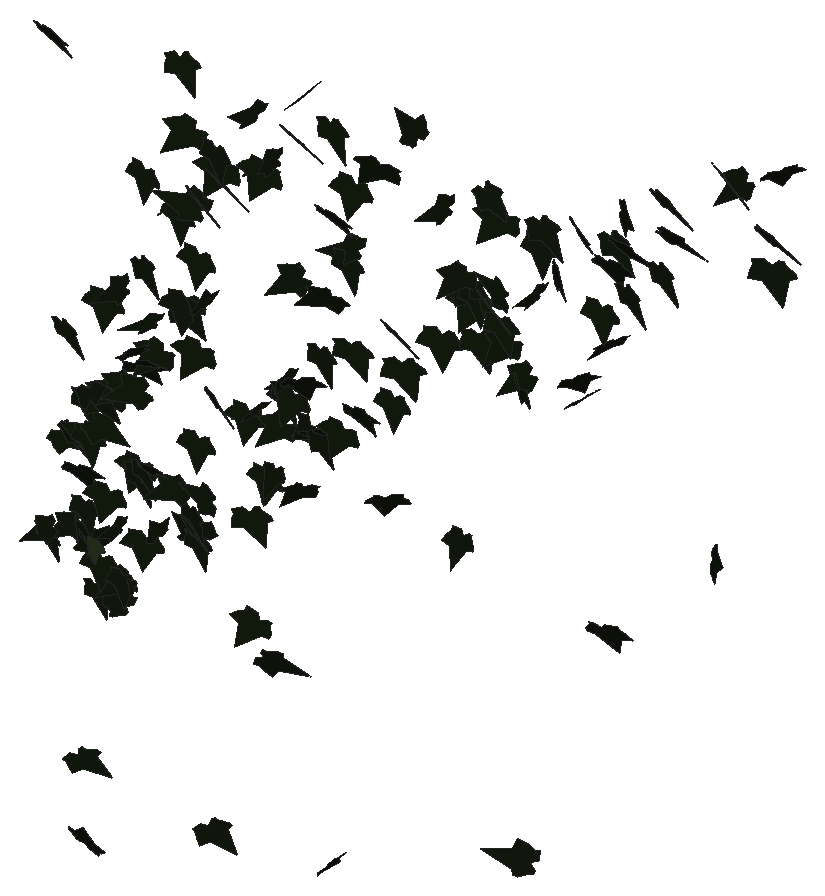
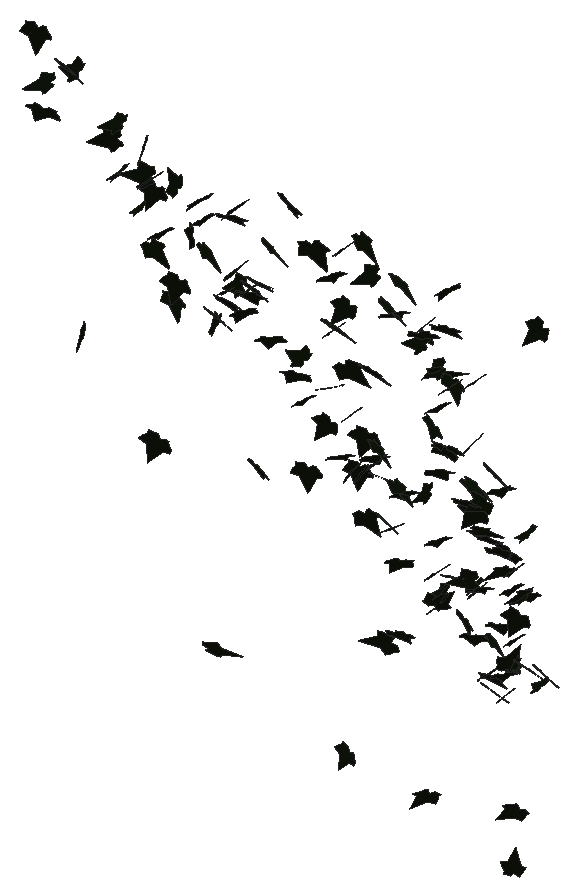
# SketchUp Ruby script. Lengths in inches.
U = 1.inch
M = Sketchup.active_model
def pt(a) = Geom::Point3d.new(a.map { |v| v * U })
def face(e, loops, mat)
  f = e.add_face(loops[0].map { |a| pt(a) })
  loops[1..].each { |l| e.add_face(l.map { |a| pt(a) }).erase! }
  f.material = f.back_material = mat if mat
  f
end
# faces: each face lists its corners as indices into pts; further lists are holes
def faces(e, pts, list, mat = nil) = list.each { |f| face(e, (f[0].is_a?(Array) ? f : [f]).map { |l| l.map { |i| pts[i] } }, mat) }
# xy, xz, yz: faces in a plane at the given z, y or x. An outline is a flat list of corners, or four numbers for a rectangle; further outlines are holes
def ring(l) = l.size == 4 ? [[l[0], l[1]], [l[2], l[1]], [l[2], l[3]], [l[0], l[3]]] : l.each_slice(2).to_a
def flat(e, list, mat, &to3) = list.each { |f| face(e, (f[0].is_a?(Array) ? f : [f]).map { |l| ring(l).map { |u, v| to3.(u, v) } }, mat) }
def xy(e, z, list, mat = nil) = flat(e, list, mat) { |x, y| [x, y, z] }
def xz(e, y, list, mat = nil) = flat(e, list, mat) { |x, z| [x, y, z] }
def yz(e, x, list, mat = nil) = flat(e, list, mat) { |y, z| [x, y, z] }
def lines(e, pts, list) = list.each { |a, b| e.add_line(pt(pts[a]), pt(pts[b])) }
# prism: a flat outline (further loops are holes) pulled along v
def prism(e, loops, v, mat = nil)
  f = face(e, loops, mat); d = Geom::Vector3d.new(v.map { |x| x * U })
  f.pushpull(f.normal.samedirection?(d) ? d.length : -d.length)
end
def box(e, o, s, mat = nil) = prism(e, [[o, [o[0] + s[0], o[1], o[2]], [o[0] + s[0], o[1] + s[1], o[2]], [o[0], o[1] + s[1], o[2]]]], [0, 0, s[2]], mat)
def at(x, y, z, deg = 0) = Geom::Transformation.translation(pt([x, y, z])) * Geom::Transformation.rotation(ORIGIN, Z_AXIS, deg.degrees)
def axes(o, x, y, z) = Geom::Transformation.new([*x, 0, *y, 0, *z, 0, *pt(o).to_a, 1])
def part(name) = M.definitions.add(name)
# library, detail: a bought-in or finely detailed component or shape, given as its bounding box
def library(name, o, s) = part(name).tap { |d| box(d.entities, o, s) }
def detail(e, o, s) = box(e.add_group.entities, o, s)
def put(e, d, t, mat = nil) = e.add_instance(d, t).tap { |i| i.material = mat if mat }
def group(e, t, mat = nil) = e.add_group.tap { |g| g.transformation = t; g.material = mat if mat }.entities
root = M.entities
M.materials.add("1026 AP 7946 SUNNY SIDE UP").color = [254, 231, 186]
M.materials.add("efeu1").color = [18, 25, 13]
M.materials.add("efeu2").color = [43, 57, 29]
c1 = part("ivyleaf_9")
p = [[1.54,2.16,1.25],[1.36,2.04,1.19],[-0.21,0.99,0.68],[-0.71,1.11,0.82],[-0.85,0.86,0.67],[-0.8,0.17,0.21],
  [-0.9,-0.01,0.1],[-0.67,-0.16,-0.02],[-0.08,-0.08,-0.05],[-0.03,-0.6,-0.4],[0.65,-0.88,-0.66],[0.83,-0.6,-0.49],
  [1.29,-0.42,-0.43],[1.8125,-0.07,-0.26],[1.21,0.44,0.15]]
faces(c1.entities,p,[[0,1,2,3,4,5,6,7,8,9,10,11,12,13,14]],"efeu1")
c2 = part("ivyleaf_10")
p = [[0,0.5,-0.03],[-0.0625,2.02,-0.43],[-0.19,2.01,-0.46],[-0.54,1.05,-0.29],[-0.52,0.625,-0.18],[-0.83,0.76,-0.28],
  [-1.16,0.64,-0.33],[-1.15,0.33,-0.24],[-0.77,-0.39,0.02],[-0.3,-0.51,0.16],[0.04,-0.48,0.23],[-0.02,2.01,-0.4375],
  [-0.06,2.01,-0.43],[0.04,-0.49,0.23],[0.67,-0.49,0.14],[1.38,0.36,-0.2],[1.375,0.51,-0.24],[0.81,0.65,-0.19],
  [0.62,0.59,-0.15],[0.6,1.09,-0.28],[0.5,1.23,-0.31]]
faces(c2.entities,p,[[0,1,2,3,4,5,6,7,8,9,10],[11,12,0,13,14,15,16,17,18,19,20]],"efeu2")
put(root,c1,axes([162.75,212.21,305.35],[-0.58936,0.16137,-0.01627],[0.00104,-0.04054,-0.41891],[-0.2551,-0.37299,0.03588]),"1026 AP 7946 SUNNY SIDE UP")
put(root,c1,axes([162.14,212.74,304.72],[0.13705,-0.36812,0.14825],[0.09896,-0.13471,-0.38942],[0.61478,0.10375,0.02964]),"1026 AP 7946 SUNNY SIDE UP")
put(root,c1,axes([162.59,212.12,327.21],[0.72573,-0.06961,-0.11126],[-0.16662,0.01892,-0.48073],[0.11334,0.47354,0.00569]),"1026 AP 7946 SUNNY SIDE UP")
put(root,c1,axes([163.57,212.73,305.6],[-0.62488,0.06034,-0.0256],[0.01594,-0.09645,-0.40326],[-0.10157,-0.38635,0.09422]),"1026 AP 7946 SUNNY SIDE UP")
put(root,c1,axes([163.01,212.68,314.14],[0.28954,-0.39286,0.03266],[0.05286,-0.02168,-0.44657],[0.61778,0.18598,0.0229]),"1026 AP 7946 SUNNY SIDE UP")
put(root,c1,axes([163.45,212.0625,309.875],[0.20026,-0.17543,-0.39382],[0.06773,0.40181,-0.17329],[0.65646,0.01206,0.13801]),"1026 AP 7946 SUNNY SIDE UP")
put(root,c1,axes([163.46,212.375,309.91],[0.3964,-0.34579,-0.08315],[-0.03922,0.07909,-0.43957],[0.55626,0.25199,0.02826]),"1026 AP 7946 SUNNY SIDE UP")
put(root,c1,axes([164,212.34,308.35],[0.58631,0.16717,-0.11588],[-0.15479,-0.0576,-0.42113],[-0.27739,0.38547,-0.00994]),"1026 AP 7946 SUNNY SIDE UP")
put(root,c1,axes([164.06,212.75,305.25],[-0.17011,-0.05183,0.39832],[-0.00754,-0.40132,-0.05911],[0.61381,-0.01929,0.10966]),"1026 AP 7946 SUNNY SIDE UP")
put(root,c1,axes([164.12,212.64,311.41],[0.07116,-0.42252,0.01072],[0.0082,-0.01232,-0.43782],[0.66463,0.04539,0.00425]),"1026 AP 7946 SUNNY SIDE UP")
put(root,c1,axes([164.55,212.67,305.04],[0.23988,0.17701,0.43607],[-0.58386,-0.21261,0.22876],[0.42127,-0.39546,0.06875]),"1026 AP 7946 SUNNY SIDE UP")
put(root,c1,axes([164.29,212.4375,291.98],[0.58875,-0.19361,0.0609],[-0.05498,0.06289,0.43272],[-0.31404,-0.37398,0.03841]),"1026 AP 7946 SUNNY SIDE UP")
put(root,c1,axes([164.26,212.46,306.8],[0.00685,-0.40946,0.00331],[-0.00226,-0.00556,-0.42188],[0.64389,0.00433,-0.00152]),"1026 AP 7946 SUNNY SIDE UP")
put(root,c1,axes([164.2,212.22,295.86],[-0.00043,-0.10164,-0.41008],[0.16643,0.38401,-0.09899],[0.62328,-0.10261,0.02615]),"1026 AP 7946 SUNNY SIDE UP")
put(root,c2,axes([164.47,212.43,305.25],[-0.5979,0.10292,-0.08941],[0.09895,-0.09591,-0.39909],[-0.18781,-0.37818,0.07436]),"1026 AP 7946 SUNNY SIDE UP")
put(root,c1,axes([164.45,212.45,310.01],[-0.05187,-0.42844,-0.01927],[-0.00576,0.0166,-0.44255],[0.67413,-0.03283,-0.00527]),"1026 AP 7946 SUNNY SIDE UP")
put(root,c1,axes([164.63,212.65,303.25],[0.13665,-0.39428,-0.00362],[-0.01065,-0.00019,-0.41588],[0.61987,0.08691,-0.00635]),"1026 AP 7946 SUNNY SIDE UP")
put(root,c1,axes([164.875,212.72,304.49],[-0.22061,-0.37732,-0.05005],[0.0449,0.03891,-0.41427],[0.59609,-0.14258,0.01268]),"1026 AP 7946 SUNNY SIDE UP")
put(root,c1,axes([165.23,212.73,307.53],[-0.46401,-0.27218,-0.08849],[0.14446,0.02407,-0.41098],[0.42413,-0.30597,0.04317]),"1026 AP 7946 SUNNY SIDE UP")
put(root,c1,axes([164.82,212.19,312.12],[-0.07422,-0.19099,-0.4167],[0.60399,0.18921,-0.13748],[0.35741,-0.3594,0.14579]),"1026 AP 7946 SUNNY SIDE UP")
put(root,c1,axes([165.22,212.57,316.13],[-0.25254,-0.41392,-0.01848],[0.01871,0.0121,-0.45727],[0.65104,-0.16091,0.00598]),"1026 AP 7946 SUNNY SIDE UP")
put(root,c1,axes([165.61,212.54,312.12],[-0.62394,-0.16568,0.05251],[-0.05191,-0.05514,-0.44159],[0.26803,-0.39637,0.03671]),"1026 AP 7946 SUNNY SIDE UP")
put(root,c1,axes([165.11,212.07,310.85],[0.2002,-0.21126,-0.37967],[0.03397,0.3863,-0.21889],[0.66545,0.04384,0.1254]),"1026 AP 7946 SUNNY SIDE UP")
put(root,c1,axes([165.9375,212.48,306.34],[-0.40557,0.31351,-0.02921],[0.01573,-0.03077,-0.41824],[-0.49498,-0.25786,0.01064]),"1026 AP 7946 SUNNY SIDE UP")
put(root,c1,axes([166.02,212.72,304.02],[-0.62871,-0.06189,0.01474],[-0.01351,-0.03988,-0.4152],[0.09909,-0.39811,0.03689]),"1026 AP 7946 SUNNY SIDE UP")
put(root,c1,axes([166.28,212.39,303.07],[-0.32578,0.27577,0.22164],[-0.34272,0.09158,-0.33911],[-0.42819,-0.28311,0.1028]),"1026 AP 7946 SUNNY SIDE UP")
put(root,c1,axes([166.24,212.3125,317.04],[-0.59695,0.22596,-0.04326],[0.02878,-0.05357,-0.45389],[-0.3606,-0.37832,0.03539]),"1026 AP 7946 SUNNY SIDE UP")
put(root,c1,axes([166.29,212.59,312.67],[-0.65712,-0.10362,0.04826],[-0.04123,-0.08803,-0.43661],[0.17439,-0.41128,0.07862]),"1026 AP 7946 SUNNY SIDE UP")
put(root,c1,axes([165.99,212.63,304.12],[-0.04526,-0.40161,0.05719],[-0.01813,-0.05711,-0.41507],[0.63775,-0.03012,-0.00774]),"1026 AP 7946 SUNNY SIDE UP")
put(root,c1,axes([167.13,212.37,312.77],[-0.55105,-0.08731,0.24483],[-0.34738,-0.09451,-0.37116],[0.19597,-0.41304,0.03053]),"1026 AP 7946 SUNNY SIDE UP")
put(root,c1,axes([166.74,212.74,309.29],[-0.36654,-0.34408,0.04983],[0.04276,-0.07843,-0.42318],[0.54511,-0.22521,0.0667]),"1026 AP 7946 SUNNY SIDE UP")
put(root,c1,axes([166.77,211.89,314.53],[0.38431,0.23383,0.29719],[0.24864,0.24521,-0.34293],[-0.52653,0.28647,0.05497]),"1026 AP 7946 SUNNY SIDE UP")
put(root,c1,axes([166.76,212.5,309.15],[0.18587,-0.43543,-0.01499],[-0.01327,0.01023,-0.46472],[0.6848,0.11838,-0.00494]),"1026 AP 7946 SUNNY SIDE UP")
put(root,c1,axes([167.51,212.57,315.84],[-0.46244,0.32052,-0.05591],[-0.12429,-0.14371,-0.41991],[-0.49632,-0.26265,0.15725]),"1026 AP 7946 SUNNY SIDE UP")
put(root,c1,axes([167.07,212.65,306.16],[-0.40083,-0.29335,-0.13842],[0.17067,0.08105,-0.39891],[0.47663,-0.27572,0.02643]),"1026 AP 7946 SUNNY SIDE UP")
put(root,c1,axes([167.01,212.22,313.99],[0.60141,0.22815,0.00998],[0.03939,-0.02567,-0.45755],[-0.35682,0.38171,-0.03369]),"1026 AP 7946 SUNNY SIDE UP")
put(root,c1,axes([166.9375,212.55,309.32],[0.22392,-0.38605,0.05819],[0.01124,-0.05987,-0.42401],[0.61389,0.14191,-0.01346]),"1026 AP 7946 SUNNY SIDE UP")
put(root,c1,axes([167.08,212.6,322.33],[-0.05954,-0.43388,0.13646],[-0.01785,-0.13444,-0.44947],[0.71424,-0.03953,0.00014]),"1026 AP 7946 SUNNY SIDE UP")
put(root,c1,axes([167.13,212.32,318.4375],[0.27111,-0.39331,-0.12837],[-0.10496,0.10423,-0.44139],[0.63913,0.18396,-0.01803]),"1026 AP 7946 SUNNY SIDE UP")
put(root,c1,axes([167.76,212.77,314.57],[-0.65416,-0.1283,-0.0039],[0.02582,-0.04294,-0.44626],[0.20014,-0.41381,0.04483]),"1026 AP 7946 SUNNY SIDE UP")
put(root,c1,axes([167.95,212.3125,306.79],[-0.05097,0.30212,0.29162],[-0.12961,0.2718,-0.30886],[-0.63608,-0.07959,0.03957]),"1026 AP 7946 SUNNY SIDE UP")
put(root,c1,axes([167.29,212.39,309.48],[0.60325,-0.10885,0.15948],[0.25712,0.0118,-0.40723],[0.15137,0.41377,0.05616]),"1026 AP 7946 SUNNY SIDE UP")
put(root,c1,axes([168.84,212.22,321.65],[-0.02985,0.45224,0.09556],[-0.05583,0.08857,-0.46468],[-0.72295,-0.02551,0.03194]),"1026 AP 7946 SUNNY SIDE UP")
put(root,c1,axes([169,212.37,309.18],[-0.60812,-0.06091,0.13941],[-0.1559,-0.17614,-0.37366],[0.17429,-0.37007,0.15219]),"1026 AP 7946 SUNNY SIDE UP")
put(root,c1,axes([168.75,212.71,327.79],[0.03832,-0.44831,-0.14776],[-0.01039,0.14073,-0.4617],[0.73884,0.02523,0.00117]),"1026 AP 7946 SUNNY SIDE UP")
put(root,c1,axes([168.89,212.43,321.33],[-0.03033,-0.44968,0.10861],[-0.00908,-0.10783,-0.46431],[0.72712,-0.0201,-0.00127]),"1026 AP 7946 SUNNY SIDE UP")
put(root,c1,axes([169.48,212.55,325.01],[-0.68642,-0.16484,0.05194],[-0.03872,-0.07875,-0.47655],[0.2687,-0.43244,0.06401]),"1026 AP 7946 SUNNY SIDE UP")
put(root,c1,axes([169.15,212.5,317.45],[-0.49248,-0.24866,-0.19676],[0.28729,0.07222,-0.40812],[0.399,-0.35891,0.051]),"1026 AP 7946 SUNNY SIDE UP")
put(root,c1,axes([169.91,212.3,321.78],[-0.27285,0.11389,0.42722],[-0.67522,-0.04973,-0.17159],[0.00561,-0.44618,0.12536]),"1026 AP 7946 SUNNY SIDE UP")
put(root,c1,axes([169.76,212.63,307.23],[0.19395,0.05103,0.40695],[-0.62285,-0.02464,0.13065],[0.06115,-0.41282,0.04005]),"1026 AP 7946 SUNNY SIDE UP")
put(root,c1,axes([169.15,212.42,317.23],[-0.16335,-0.20864,-0.38843],[0.59578,0.13823,-0.18612],[0.31932,-0.36463,0.14856]),"1026 AP 7946 SUNNY SIDE UP")
put(root,c1,axes([169.31,212.625,308.22],[0.18103,-0.39069,0.08867],[0.02297,-0.08771,-0.41997],[0.6294,0.11557,-0.01018]),"1026 AP 7946 SUNNY SIDE UP")
put(root,c1,axes([169.37,212.22,307.97],[0.49828,-0.28506,-0.02212],[-0.05388,-0.00847,-0.43813],[0.44608,0.3174,-0.02821]),"1026 AP 7946 SUNNY SIDE UP")
put(root,c1,axes([169.61,212.71,311.39],[-0.17906,-0.41076,0.00668],[0.01596,-0.01196,-0.43899],[0.64584,-0.11359,0.0127]),"1026 AP 7946 SUNNY SIDE UP")
put(root,c1,axes([169.93,212.41,315.57],[-0.50569,-0.30652,0.01908],[0.01308,-0.03801,-0.45663],[0.48284,-0.31999,0.03235]),"1026 AP 7946 SUNNY SIDE UP")
put(root,c1,axes([169.63,212.63,307.11],[0.07832,-0.41116,0.04099],[0.00254,-0.04224,-0.4269],[0.64989,0.04972,-0.00327]),"1026 AP 7946 SUNNY SIDE UP")
put(root,c1,axes([169.57,212.37,322.33],[0.60364,-0.2601,-0.06605],[-0.08469,0.03217,-0.47751],[0.41206,0.38764,-0.00138]),"1026 AP 7946 SUNNY SIDE UP")
put(root,c1,axes([170.13,212.74,308.86],[-0.04906,-0.41259,-0.06283],[-0.01117,-0.05827,0.42591],[-0.65518,0.03189,-0.00256]),"1026 AP 7946 SUNNY SIDE UP")
put(root,c1,axes([169.86,212.43,319.66],[-0.15812,-0.44032,0.07636],[0.00365,-0.07905,-0.46532],[0.70276,-0.09866,0.0196]),"1026 AP 7946 SUNNY SIDE UP")
put(root,c1,axes([170.57,211.76,317.98],[0.09648,0.31108,0.33552],[-0.03983,0.3288,-0.31844],[-0.70504,0.024,0.0639]),"1026 AP 7946 SUNNY SIDE UP")
put(root,c1,axes([170.39,212.47,294.79],[-0.01601,-0.2121,-0.40014],[0.04284,0.38627,-0.21646],[0.69288,-0.02879,0.00414]),"1026 AP 7946 SUNNY SIDE UP")
put(root,c1,axes([170.55,212.24,313.9375],[0.52024,-0.29178,-0.0417],[-0.07705,0.003,-0.45339],[0.45639,0.33312,-0.029]),"1026 AP 7946 SUNNY SIDE UP")
put(root,c1,axes([170.6875,212.43,324.61],[0.05953,-0.46122,0.08895],[-0.01522,-0.08999,-0.47696],[0.73843,0.03533,-0.017]),"1026 AP 7946 SUNNY SIDE UP")
put(root,c1,axes([171.05,212.45,324],[-0.57183,-0.28638,-0.02261],[0.05335,-0.01031,-0.47599],[0.44827,-0.36409,0.02781]),"1026 AP 7946 SUNNY SIDE UP")
put(root,c1,axes([170.77,212.35,323.4375],[0.47725,-0.3256,0.15661],[0.2025,-0.08979,-0.45796],[0.52881,0.32823,0.03403]),"1026 AP 7946 SUNNY SIDE UP")
put(root,c1,axes([172.11,212.67,313.5],[-0.2765,-0.39618,-0.00043],[0.04015,-0.01333,-0.44563],[0.62166,-0.17535,0.02859]),"1026 AP 7946 SUNNY SIDE UP")
put(root,c1,axes([172.67,212.38,326.87],[-0.37102,0.39801,0.07081],[-0.12903,0.02807,-0.47304],[-0.62125,-0.24353,0.05595]),"1026 AP 7946 SUNNY SIDE UP")
put(root,c1,axes([172.71,212.49,313.84],[-0.31177,0.37957,-0.05425],[-0.07761,-0.08645,-0.43329],[-0.59801,-0.18667,0.08452]),"1026 AP 7946 SUNNY SIDE UP")
put(root,c1,axes([172.51,212.72,304.47],[-0.59381,-0.19962,-0.0098],[0.04495,-0.03625,-0.43778],[0.31093,-0.37599,0.04457]),"1026 AP 7946 SUNNY SIDE UP")
put(root,c1,axes([172.24,212.62,309.11],[-0.15295,-0.32482,-0.26201],[0.15784,0.23287,-0.3471],[0.62735,-0.13778,0.02345]),"1026 AP 7946 SUNNY SIDE UP")
put(root,c1,axes([173.09,212.46,324.55],[-0.4226,-0.3763,0.08641],[0.01546,-0.11144,-0.4713],[0.60676,-0.25925,0.07219]),"1026 AP 7946 SUNNY SIDE UP")
put(root,c1,axes([172.97,212.75,310.97],[-0.17975,-0.39371,0.1036],[0.04524,-0.11433,-0.41881],[0.63822,-0.10278,0.05886]),"1026 AP 7946 SUNNY SIDE UP")
put(root,c1,axes([173.56,212.47,325.13],[-0.57076,0.29209,-0.07701],[0.03058,-0.09662,-0.47624],[-0.47374,-0.35814,0.06204]),"1026 AP 7946 SUNNY SIDE UP")
put(root,c1,axes([173.33,212.7,311.33],[-0.50913,-0.07442,-0.27514],[0.43415,-0.11682,-0.31249],[-0.03184,-0.40287,0.1388]),"1026 AP 7946 SUNNY SIDE UP")
put(root,c1,axes([173.37,212.19,303.33],[0.17222,0.07093,-0.42669],[0.42067,0.31883,0.13087],[0.51033,-0.28675,0.03611]),"1026 AP 7946 SUNNY SIDE UP")
put(root,c1,axes([174.11,212.38,313.79],[-0.67042,-0.10578,-0.03602],[0.1111,-0.15249,-0.42052],[0.13506,-0.39964,0.16714]),"1026 AP 7946 SUNNY SIDE UP")
put(root,c1,axes([174.27,212.375,315.78],[-0.36511,0.37092,0.00012],[-0.02676,-0.013,-0.45036],[-0.58264,-0.23184,0.02061]),"1026 AP 7946 SUNNY SIDE UP")
put(root,c1,axes([173.73,212.75,315],[0.14819,-0.42503,0.01787],[0.00438,-0.01962,-0.44862],[0.66903,0.09428,-0.00102]),"1026 AP 7946 SUNNY SIDE UP")
put(root,c1,axes([174.34,212.61,315.02],[-0.38586,-0.35945,0.02173],[0.02277,-0.03781,-0.44728],[0.56591,-0.24357,0.03281]),"1026 AP 7946 SUNNY SIDE UP")
put(root,c1,axes([174.83,212.43,320.45],[-0.71096,0.05789,0.01207],[-0.0278,-0.049,-0.46696],[-0.08851,-0.44963,0.04974]),"1026 AP 7946 SUNNY SIDE UP")
put(root,c1,axes([174.82,212.58,311.17],[0.00987,0.29557,-0.31881],[-0.07229,-0.30893,-0.30509],[-0.67093,0.03764,0.02818]),"1026 AP 7946 SUNNY SIDE UP")
put(root,c1,axes([174.25,212.41,326.66],[0.66866,-0.20076,0.00525],[0.03076,0.02686,-0.48313],[0.31433,0.42445,0.0361]),"1026 AP 7946 SUNNY SIDE UP")
put(root,c1,axes([175.18,212.49,328.7],[-0.31293,0.40696,-0.15753],[0.06585,-0.15199,-0.46672],[-0.6817,-0.20149,0.02723]),"1026 AP 7946 SUNNY SIDE UP")
put(root,c1,axes([174.95,212.18,316.06],[0.47296,0.30901,-0.08348],[-0.05602,-0.08057,-0.44364],[-0.49989,0.30139,-0.02927]),"1026 AP 7946 SUNNY SIDE UP")
put(root,c1,axes([174.91,212.88,313.82],[0.18608,-0.22379,-0.35743],[0.29881,-0.28941,0.25834],[-0.57445,-0.22303,0.0186]),"1026 AP 7946 SUNNY SIDE UP")
put(root,c1,axes([175.37,212.36,313.89],[0.29252,0.38184,-0.05795],[-0.07197,-0.04259,-0.43722],[-0.60312,0.19028,0.02407]),"1026 AP 7946 SUNNY SIDE UP")
put(root,c1,axes([176.24,212.47,320.11],[0.02364,0.17531,-0.43494],[-0.43895,-0.33219,-0.15393],[-0.57104,0.26261,0.10032]),"1026 AP 7946 SUNNY SIDE UP")
put(root,c1,axes([175.61,212.5,313.79],[0.2613,-0.37194,-0.17017],[-0.15143,0.13508,-0.41771],[0.62037,0.18963,-0.03028]),"1026 AP 7946 SUNNY SIDE UP")
put(root,c1,axes([175.63,212.67,317.36],[0.11901,-0.43848,0.00236],[-0.00167,-0.00504,-0.45842],[0.68951,0.07567,-0.00152]),"1026 AP 7946 SUNNY SIDE UP")
put(root,c1,axes([176.33,212.21,295.26],[0.14648,0.35506,0.2527],[0.12552,0.23034,-0.37647],[-0.66503,0.12168,-0.0154]),"1026 AP 7946 SUNNY SIDE UP")
put(root,c1,axes([176.25,212.29,323.87],[0.70313,0.00976,-0.11709],[-0.17947,0.03921,-0.45867],[0.00038,0.45973,0.04432]),"1026 AP 7946 SUNNY SIDE UP")
put(root,c1,axes([176.34,212.45,327.66],[0.1407,-0.46955,-0.04041],[-0.01356,0.03558,-0.49223],[0.74044,0.08988,-0.00133]),"1026 AP 7946 SUNNY SIDE UP")
put(root,c1,axes([176.68,212.74,314.27],[-0.38341,-0.3502,0.07718],[0.03479,-0.10752,-0.43277],[0.5627,-0.23197,0.07934]),"1026 AP 7946 SUNNY SIDE UP")
put(root,c1,axes([177.42,212.58,322.5],[-0.53767,0.29514,0.10478],[-0.25659,-0.04305,-0.44402],[-0.41746,-0.35367,0.13796]),"1026 AP 7946 SUNNY SIDE UP")
put(root,c1,axes([177.16,212.43,322.1],[0.0412,-0.45722,0.04575],[-0.00006,-0.04708,-0.47207],[0.72273,0.02606,-0.00265]),"1026 AP 7946 SUNNY SIDE UP")
put(root,c1,axes([177.48,212.4375,325.42],[-0.2846,-0.4314,0.0317],[0.00701,-0.03787,-0.4818],[0.68031,-0.18008,0.01823]),"1026 AP 7946 SUNNY SIDE UP")
put(root,c1,axes([177.37,212.4,318.34],[-0.04722,-0.44196,-0.05212],[0.23465,0.03538,-0.43078],[0.65848,-0.0443,0.14977]),"1026 AP 7946 SUNNY SIDE UP")
put(root,c1,axes([177.78,212.09,315.81],[0.66366,0.03544,-0.0996],[-0.14722,-0.03975,-0.4354],[-0.06811,0.43121,-0.02939]),"1026 AP 7946 SUNNY SIDE UP")
put(root,c1,axes([178.82,212.28,326.85],[0.3173,0.18192,-0.40383],[-0.43378,-0.28026,-0.28119],[-0.52496,0.34154,-0.01173]),"1026 AP 7946 SUNNY SIDE UP")
put(root,c1,axes([179.1875,212.22,312.4],[0.32183,0.3571,-0.14938],[-0.09059,-0.1363,-0.42447],[-0.60044,0.21196,-0.01602]),"1026 AP 7946 SUNNY SIDE UP")
put(root,c1,axes([179.44,212.4,316.75],[-0.10511,-0.43286,0.06161],[-0.00551,-0.06245,-0.45154],[0.68762,-0.06667,0.0058]),"1026 AP 7946 SUNNY SIDE UP")
put(root,c1,axes([179.25,212.62,319.54],[0.23194,-0.32968,0.27807],[0.29474,-0.20846,-0.36651],[0.60375,0.22842,0.0721]),"1026 AP 7946 SUNNY SIDE UP")
put(root,c1,axes([179.8,212.48,318.36],[-0.26134,-0.31631,-0.2724],[0.333,0.17692,-0.35656],[0.55407,-0.25552,0.08582]),"1026 AP 7946 SUNNY SIDE UP")
put(root,c1,axes([180.7,212.18,328.81],[-0.09111,0.19973,0.44828],[-0.34135,0.37844,-0.20706],[-0.6692,-0.22023,0.04459]),"1026 AP 7946 SUNNY SIDE UP")
put(root,c1,axes([181.97,212.46,325.99],[-0.56098,0.30848,-0.02304],[-0.00751,-0.04229,-0.48478],[-0.48647,-0.35507,0.03405]),"1026 AP 7946 SUNNY SIDE UP")
put(root,c1,axes([181.53,212.7,320.14],[-0.32128,-0.37703,-0.13988],[0.14322,0.10227,-0.4401],[0.61245,-0.22169,0.02954]),"1026 AP 7946 SUNNY SIDE UP")
put(root,c1,axes([182.52,212.71,311.66],[-0.56336,-0.0192,-0.28216],[0.43021,-0.06036,-0.36485],[-0.03391,-0.44685,0.05875]),"1026 AP 7946 SUNNY SIDE UP")
put(root,c1,axes([182.71,212.6,323.31],[-0.6825,-0.1158,-0.1155],[0.23953,-0.19403,-0.4046],[0.08059,-0.40395,0.22435]),"1026 AP 7946 SUNNY SIDE UP")
put(root,c1,axes([183.09,212.37,322.6],[-0.67267,0.11094,-0.15813],[-0.21579,0.08194,0.45367],[0.20639,0.44727,-0.04103]),"1026 AP 7946 SUNNY SIDE UP")
put(root,c1,axes([183.3,212.59,322.35],[-0.58899,-0.25436,-0.07316],[0.13905,-0.00731,-0.46303],[0.39064,-0.38092,0.05452]),"1026 AP 7946 SUNNY SIDE UP")
put(root,c1,axes([183.15,212.72,322.63],[0.01287,-0.45572,0.04381],[-0.00007,-0.04512,-0.46982],[0.72008,0.00814,-0.00083]),"1026 AP 7946 SUNNY SIDE UP")
put(root,c1,axes([183.61,212.37,320.98],[-0.08907,-0.41031,-0.17578],[0.05893,0.16463,-0.42552],[0.69484,-0.06656,0.01356]),"1026 AP 7946 SUNNY SIDE UP")
put(root,c1,axes([183.75,212.47,322.62],[0.50195,-0.30049,0.12453],[0.08687,-0.11912,-0.44973],[0.50284,0.32053,-0.04662]),"1026 AP 7946 SUNNY SIDE UP")
put(root,c1,axes([184.05,212.26,327.57],[0.28709,-0.37947,-0.2445],[-0.07848,0.23514,-0.42941],[0.69758,0.18263,0.05232]),"1026 AP 7946 SUNNY SIDE UP")
put(root,c1,axes([184.57,212.62,322.96],[0.01252,-0.46013,0.03649],[-0.00755,0.03796,0.4743],[-0.72594,-0.00833,-0.0043]),"1026 AP 7946 SUNNY SIDE UP")
put(root,c1,axes([184.83,212.4,326.66],[-0.66384,-0.22136,0.01006],[0.0542,-0.08901,-0.4818],[0.34425,-0.41284,0.09526]),"1026 AP 7946 SUNNY SIDE UP")
put(root,c1,axes([185.08,212.45,321.26],[-0.69803,-0.03624,-0.08419],[0.13388,-0.0486,-0.45569],[0.04187,-0.44872,0.05348]),"1026 AP 7946 SUNNY SIDE UP")
put(root,c1,axes([184.68,212.38,322.02],[0.00275,-0.44979,-0.0166],[0.06629,0.01367,-0.46125],[0.70446,0.00047,0.04347]),"1026 AP 7946 SUNNY SIDE UP")
put(root,c1,axes([185.92,212.51,298.67],[-0.41376,0.07255,0.38147],[-0.58175,0.03649,-0.27832],[-0.11327,-0.45246,0.03599]),"1026 AP 7946 SUNNY SIDE UP")
put(root,c1,axes([185.98,212.41,320.1],[-0.68556,0.09621,-0.07286],[0.08701,-0.07675,-0.45592],[-0.16695,-0.43506,0.06157]),"1026 AP 7946 SUNNY SIDE UP")
put(root,c1,axes([185.53,212.53,319.47],[0.31271,-0.18316,-0.37726],[0.48239,-0.20123,0.27493],[-0.42419,-0.36387,0.03454]),"1026 AP 7946 SUNNY SIDE UP")
put(root,c1,axes([186.63,212.22,323.93],[-0.40436,0.37512,-0.05314],[0.01596,-0.05807,-0.46821],[-0.59564,-0.25621,0.02353]),"1026 AP 7946 SUNNY SIDE UP")
put(root,c1,axes([186.43,212.66,325.98],[-0.05942,-0.46605,0.03418],[-0.02235,-0.03478,-0.48176],[0.73465,-0.03875,-0.01189]),"1026 AP 7946 SUNNY SIDE UP")
put(root,c1,axes([186.71,212.31,327.05],[0.17826,-0.43889,-0.17134],[0.00608,0.16942,-0.46385],[0.7366,0.10482,0.0453]),"1026 AP 7946 SUNNY SIDE UP")
put(root,c1,axes([186.97,212.84,324.875],[0.05841,-0.06312,-0.46851],[0.68329,-0.14137,0.056],[-0.23135,-0.43347,0.0471]),"1026 AP 7946 SUNNY SIDE UP")
put(root,c1,axes([188.71,212.35,320.07],[0.00137,0.45689,0.02827],[-0.0382,0.02486,-0.46988],[-0.71847,-0.00045,0.02504]),"1026 AP 7946 SUNNY SIDE UP")
put(root,c1,axes([188.59,212.02,321],[0.32579,0.40945,0.01778],[0.04522,0.00215,-0.47205],[-0.64266,0.20772,-0.02421]),"1026 AP 7946 SUNNY SIDE UP")
put(root,c1,axes([188.35,212.47,327.29],[0.47507,-0.17282,-0.33908],[0.49889,-0.09876,0.35394],[-0.30201,-0.43499,0.05128]),"1026 AP 7946 SUNNY SIDE UP")
put(root,c1,axes([189.39,212.67,324.1],[-0.09029,-0.45919,0.02026],[0.00434,-0.02279,-0.47684],[0.72287,-0.05722,0.00539]),"1026 AP 7946 SUNNY SIDE UP")
put(root,c1,axes([190.13,212.5,323],[-0.18326,0.3769,-0.25092],[-0.00979,-0.25514,-0.40164],[-0.70738,-0.09411,0.07056]),"1026 AP 7946 SUNNY SIDE UP")
put(root,c1,axes([189.86,212.1875,310.46],[0.65192,0.18044,-0.12177],[-0.14188,-0.08996,-0.46403],[-0.30905,0.42192,-0.04384]),"1026 AP 7946 SUNNY SIDE UP")
put(root,c1,axes([190.05,212.24,326.55],[0.65373,0.11046,-0.17397],[-0.25224,-0.05604,-0.44331],[-0.19383,0.44546,-0.00983]),"1026 AP 7946 SUNNY SIDE UP")
put(root,c1,axes([189.95,212.6,327.4],[0.22425,-0.42114,-0.15163],[-0.01011,0.15007,-0.45532],[0.70017,0.13704,0.04199]),"1026 AP 7946 SUNNY SIDE UP")
put(root,c1,axes([190.93,212.01,329.17],[0.32072,-0.14405,-0.41938],[-0.50973,0.24498,-0.25571],[0.44673,0.38294,0.0093]),"1026 AP 7946 SUNNY SIDE UP")
put(root,c1,axes([190.375,212.47,327.28],[0.58937,-0.17703,0.24334],[0.35868,-0.07114,-0.42643],[0.29658,0.43784,0.03215]),"1026 AP 7946 SUNNY SIDE UP")
put(root,c1,axes([190.66,212.6,325.36],[0.31553,-0.41972,-0.01097],[-0.01665,0.0041,-0.47918],[0.65989,0.2008,-0.00685]),"1026 AP 7946 SUNNY SIDE UP")
put(root,c1,axes([192.31,212.54,326.92],[0.28795,-0.43105,-0.03884],[-0.02708,0.03099,-0.48228],[0.67951,0.1839,-0.00276]),"1026 AP 7946 SUNNY SIDE UP")
put(root,c1,axes([192.26,212.62,330.08],[0.50413,-0.34045,0.05133],[0.12708,0.00564,-0.47744],[0.52636,0.32471,0.06611]),"1026 AP 7946 SUNNY SIDE UP")
put(root,c1,axes([192.83,212.3,328.74],[0.66332,-0.10823,0.17718],[0.26455,-0.03874,-0.44887],[0.18065,0.45415,0.00676]),"1026 AP 7946 SUNNY SIDE UP")
put(root,c1,axes([195.49,211.88,315.56],[0.16419,-0.0416,-0.48027],[-0.56354,0.29973,-0.10855],[0.47277,0.37173,0.0374]),"1026 AP 7946 SUNNY SIDE UP")
put(root,c1,axes([195.49,212.45,332.1875],[0.37969,-0.34564,0.23785],[0.2014,-0.19453,-0.43546],[0.62358,0.27328,-0.00418]),"1026 AP 7946 SUNNY SIDE UP")
put(root,c1,axes([196.57,212.44,332.28],[-0.71798,0.09952,-0.09969],[0.13384,-0.0645,-0.47968],[-0.1732,-0.46239,0.04257]),"1026 AP 7946 SUNNY SIDE UP")
put(root,c1,axes([197.89,212.49,328.98],[-0.40228,-0.2508,-0.33324],[0.40951,0.19237,-0.36634],[0.49421,-0.36354,0.03231]),"1026 AP 7946 SUNNY SIDE UP")
put(root,c1,axes([197.71,212.16,330.6],[0.62224,-0.27103,0.00249],[0.08761,0.07449,-0.48432],[0.41711,0.38867,0.09802]),"1026 AP 7946 SUNNY SIDE UP")
put(root,c1,axes([198.66,212.02,333.64],[0.23201,0.45731,-0.0324],[-0.00205,-0.03534,-0.49514],[-0.72106,0.14724,-0.00902]),"1026 AP 7946 SUNNY SIDE UP")
